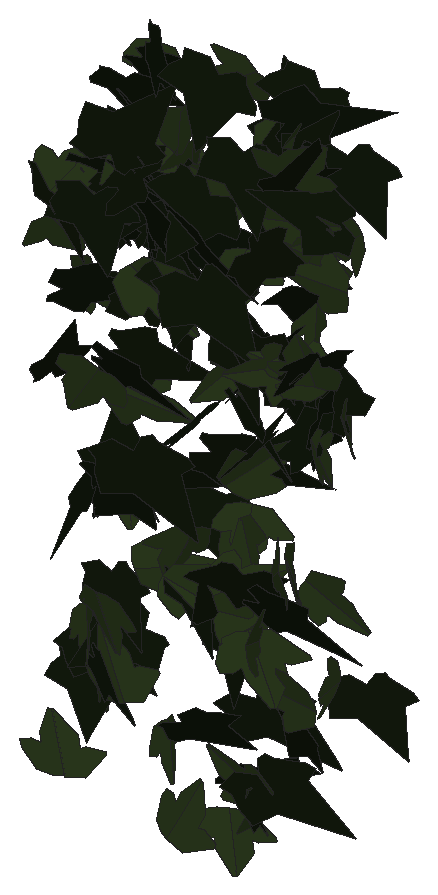
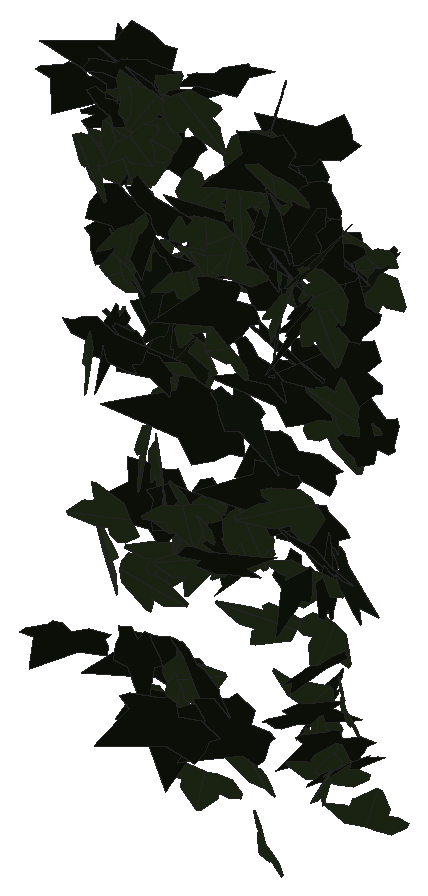
# SketchUp Ruby script. Lengths in inches.
U = 1.inch
M = Sketchup.active_model
def pt(a) = Geom::Point3d.new(a.map { |v| v * U })
def face(e, loops, mat)
  f = e.add_face(loops[0].map { |a| pt(a) })
  loops[1..].each { |l| e.add_face(l.map { |a| pt(a) }).erase! }
  f.material = f.back_material = mat if mat
  f
end
# faces: each face lists its corners as indices into pts; further lists are holes
def faces(e, pts, list, mat = nil) = list.each { |f| face(e, (f[0].is_a?(Array) ? f : [f]).map { |l| l.map { |i| pts[i] } }, mat) }
# xy, xz, yz: faces in a plane at the given z, y or x. An outline is a flat list of corners, or four numbers for a rectangle; further outlines are holes
def ring(l) = l.size == 4 ? [[l[0], l[1]], [l[2], l[1]], [l[2], l[3]], [l[0], l[3]]] : l.each_slice(2).to_a
def flat(e, list, mat, &to3) = list.each { |f| face(e, (f[0].is_a?(Array) ? f : [f]).map { |l| ring(l).map { |u, v| to3.(u, v) } }, mat) }
def xy(e, z, list, mat = nil) = flat(e, list, mat) { |x, y| [x, y, z] }
def xz(e, y, list, mat = nil) = flat(e, list, mat) { |x, z| [x, y, z] }
def yz(e, x, list, mat = nil) = flat(e, list, mat) { |y, z| [x, y, z] }
def lines(e, pts, list) = list.each { |a, b| e.add_line(pt(pts[a]), pt(pts[b])) }
# prism: a flat outline (further loops are holes) pulled along v
def prism(e, loops, v, mat = nil)
  f = face(e, loops, mat); d = Geom::Vector3d.new(v.map { |x| x * U })
  f.pushpull(f.normal.samedirection?(d) ? d.length : -d.length)
end
def box(e, o, s, mat = nil) = prism(e, [[o, [o[0] + s[0], o[1], o[2]], [o[0] + s[0], o[1] + s[1], o[2]], [o[0], o[1] + s[1], o[2]]]], [0, 0, s[2]], mat)
def at(x, y, z, deg = 0) = Geom::Transformation.translation(pt([x, y, z])) * Geom::Transformation.rotation(ORIGIN, Z_AXIS, deg.degrees)
def axes(o, x, y, z) = Geom::Transformation.new([*x, 0, *y, 0, *z, 0, *pt(o).to_a, 1])
def part(name) = M.definitions.add(name)
# library, detail: a bought-in or finely detailed component or shape, given as its bounding box
def library(name, o, s) = part(name).tap { |d| box(d.entities, o, s) }
def detail(e, o, s) = box(e.add_group.entities, o, s)
def put(e, d, t, mat = nil) = e.add_instance(d, t).tap { |i| i.material = mat if mat }
def group(e, t, mat = nil) = e.add_group.tap { |g| g.transformation = t; g.material = mat if mat }.entities
root = M.entities
M.materials.add("1026 AP 7946 SUNNY SIDE UP").color = [254, 231, 186]
M.materials.add("efeu1").color = [18, 25, 13]
M.materials.add("efeu2").color = [43, 57, 29]
c1 = part("ivyleaf_9")
p = [[1.54,2.16,1.25],[1.36,2.04,1.19],[-0.21,0.99,0.68],[-0.71,1.11,0.82],[-0.85,0.86,0.67],[-0.8,0.17,0.21],
  [-0.9,-0.01,0.1],[-0.67,-0.16,-0.02],[-0.08,-0.08,-0.05],[-0.03,-0.6,-0.4],[0.65,-0.88,-0.66],[0.83,-0.6,-0.49],
  [1.29,-0.42,-0.43],[1.8125,-0.07,-0.26],[1.21,0.44,0.15]]
faces(c1.entities,p,[[0,1,2,3,4,5,6,7,8,9,10,11,12,13,14]],"efeu1")
c2 = part("ivyleaf_10")
p = [[0,0.5,-0.03],[-0.0625,2.02,-0.43],[-0.19,2.01,-0.46],[-0.54,1.05,-0.29],[-0.52,0.625,-0.18],[-0.83,0.76,-0.28],
  [-1.16,0.64,-0.33],[-1.15,0.33,-0.24],[-0.77,-0.39,0.02],[-0.3,-0.51,0.16],[0.04,-0.48,0.23],[-0.02,2.01,-0.4375],
  [-0.06,2.01,-0.43],[0.04,-0.49,0.23],[0.67,-0.49,0.14],[1.38,0.36,-0.2],[1.375,0.51,-0.24],[0.81,0.65,-0.19],
  [0.62,0.59,-0.15],[0.6,1.09,-0.28],[0.5,1.23,-0.31]]
faces(c2.entities,p,[[0,1,2,3,4,5,6,7,8,9,10],[11,12,0,13,14,15,16,17,18,19,20]],"efeu2")
put(root,c1,axes([131.8,211.0625,274.17],[0.20977,0.25141,0.15948],[-0.19832,-0.10338,0.28698],[0.41845,-0.17502,0.05607]),"1026 AP 7946 SUNNY SIDE UP")
put(root,c2,axes([131.75,212.14,277.14],[-0.34587,0.07904,-0.20582],[0.25115,-0.13201,-0.23521],[-0.22694,-0.26655,0.05338]),"1026 AP 7946 SUNNY SIDE UP")
put(root,c1,axes([131.69,211.18,276.95],[0.1745,-0.32235,0.06334],[0.00781,-0.06517,-0.35119],[0.51649,0.10989,-0.01609]),"1026 AP 7946 SUNNY SIDE UP")
put(root,c2,axes([131.96,211.03,268.16],[0.45955,0.14826,0.03924],[-0.07352,0.01018,0.33625],[0.22885,-0.29445,0.02922]),"1026 AP 7946 SUNNY SIDE UP")
put(root,c2,axes([131.58,211.93,275.12],[0.00813,-0.00522,0.33783],[0.50626,-0.06254,-0.00662],[0.09847,0.32198,0.00615]),"1026 AP 7946 SUNNY SIDE UP")
put(root,c2,axes([131.96,210.88,276.61],[-0.22401,-0.24818,-0.19154],[0.17393,0.14883,-0.29333],[0.45411,-0.17943,0.01786]),"1026 AP 7946 SUNNY SIDE UP")
put(root,c1,axes([131.93,211.68,269.27],[-0.11331,-0.31358,0.02304],[0.00257,-0.02514,-0.33154],[0.49453,-0.07172,0.007]),"1026 AP 7946 SUNNY SIDE UP")
put(root,c2,axes([132.12,211.84,276.39],[-0.2045,-0.2943,0.06603],[-0.01394,-0.06786,-0.3313],[0.47397,-0.12898,0.01875]),"1026 AP 7946 SUNNY SIDE UP")
put(root,c1,axes([132.0625,211.5,272.28],[-0.34976,0.10596,-0.2904],[0.35323,-0.17612,-0.25131],[-0.31669,-0.31346,0.04042]),"1026 AP 7946 SUNNY SIDE UP")
put(root,c2,axes([132.07,211.7,269.17],[0.13469,-0.04751,-0.32807],[0.02732,0.32947,-0.04394],[0.50512,-0.00515,0.08986]),"1026 AP 7946 SUNNY SIDE UP")
put(root,c1,axes([131.98,211.6875,276.33],[0.50369,-0.15543,0.11191],[-0.12676,0.08328,0.36519],[-0.27076,-0.32813,0.03721]),"1026 AP 7946 SUNNY SIDE UP")
put(root,c1,axes([132,211.89,271.93],[0.04023,0.15172,0.30183],[-0.1497,-0.27707,0.15521],[0.49546,-0.09603,0.02239]),"1026 AP 7946 SUNNY SIDE UP")
put(root,c2,axes([131.875,211.1,277.09],[0.43761,0.04456,-0.16717],[0.22882,0.09467,0.28402],[0.13361,-0.30807,0.06109]),"1026 AP 7946 SUNNY SIDE UP")
put(root,c2,axes([132.11,211.7,269.12],[0.42989,0.18068,0.01962],[-0.0551,0.02054,0.33563],[0.28015,-0.27322,0.03591]),"1026 AP 7946 SUNNY SIDE UP")
put(root,c2,axes([131.88,211.59,270.18],[0.24733,-0.12321,0.26108],[0.29901,-0.16887,-0.20658],[0.32834,0.24659,-0.00854]),"1026 AP 7946 SUNNY SIDE UP")
put(root,c1,axes([132.18,212.23,277.25],[0.12672,-0.30585,-0.08111],[0.0579,-0.06981,0.32494],[-0.49254,-0.0869,0.01733]),"1026 AP 7946 SUNNY SIDE UP")
put(root,c1,axes([131.89,211.75,269.78],[0.07443,-0.18799,-0.26741],[0.09615,0.26182,-0.18308],[0.4933,-0.02267,0.07603]),"1026 AP 7946 SUNNY SIDE UP")
put(root,c1,axes([131.9,211.23,275.375],[0.28457,0.11751,0.29411],[0.41075,0.11664,-0.21989],[-0.25691,0.31666,-0.02579]),"1026 AP 7946 SUNNY SIDE UP")
put(root,c1,axes([132.42,211.77,272.5625],[-0.46411,0.12535,-0.06044],[-0.0735,0.04155,0.32998],[0.20534,0.29819,-0.01849]),"1026 AP 7946 SUNNY SIDE UP")
put(root,c1,axes([132.33,211.85,277.1],[0.34853,0.00144,0.2401],[-0.35863,0.06745,0.22344],[-0.07533,-0.31447,0.0471]),"1026 AP 7946 SUNNY SIDE UP")
put(root,c2,axes([132.54,211.03,274.33],[-0.49408,-0.03623,0.16001],[-0.23489,-0.05466,-0.32436],[0.08877,-0.34632,0.03236]),"1026 AP 7946 SUNNY SIDE UP")
put(root,c2,axes([132.35,211.7,269.33],[-0.4231,0.19063,0.03773],[0.06763,-0.0006,0.3388],[0.29732,0.27142,-0.02337]),"1026 AP 7946 SUNNY SIDE UP")
put(root,c1,axes([132.24,211.99,276.53],[0.23175,-0.20854,-0.26088],[-0.22103,0.20925,-0.26182],[0.46448,0.20363,0.00558]),"1026 AP 7946 SUNNY SIDE UP")
put(root,c1,axes([132.01,212.22,277.96],[0.36104,-0.19128,0.11563],[0.11208,-0.09098,-0.30751],[0.33113,0.23935,-0.02198]),"1026 AP 7946 SUNNY SIDE UP")
put(root,c1,axes([132.4375,212.08,276.42],[-0.1331,-0.1509,0.27183],[-0.19324,-0.2345,-0.17957],[0.43843,-0.14917,0.00338]),"1026 AP 7946 SUNNY SIDE UP")
put(root,c1,axes([132.39,211.92,278.47],[0.43253,0.13542,-0.12739],[-0.1516,-0.08445,-0.31476],[-0.24625,0.28985,-0.02998]),"1026 AP 7946 SUNNY SIDE UP")
put(root,c1,axes([132.6,211.95,270.02],[-0.36249,-0.19367,0.19789],[-0.19346,-0.15224,-0.30937],[0.38417,-0.25941,0.03093]),"1026 AP 7946 SUNNY SIDE UP")
put(root,c1,axes([132.26,211.76,270.83],[0.05408,-0.31384,-0.08522],[-0.00413,0.08112,-0.32472],[0.50961,0.03396,0.00641]),"1026 AP 7946 SUNNY SIDE UP")
put(root,c1,axes([132.43,211.96,272.34],[0.37578,-0.08418,-0.21747],[-0.31577,0.06371,-0.2606],[0.16581,0.31211,-0.00343]),"1026 AP 7946 SUNNY SIDE UP")
put(root,c2,axes([132.31,211.91,272.31],[0.47828,0.0842,0.08091],[0.1293,-0.0055,-0.32403],[-0.12599,0.31398,-0.02541]),"1026 AP 7946 SUNNY SIDE UP")
put(root,c1,axes([132.08,211.36,277.11],[0.40822,0.02408,0.25176],[0.38563,-0.03881,-0.26485],[0.01449,0.35433,-0.04401]),"1026 AP 7946 SUNNY SIDE UP")
put(root,c1,axes([132.6,212.0625,277.875],[0.04334,0.1272,0.34532],[0.11939,0.32576,-0.13216],[-0.54987,0.08075,-0.00148]),"1026 AP 7946 SUNNY SIDE UP")
put(root,c2,axes([132.55,212.15,276.6875],[-0.06651,0.30731,0.06583],[-0.03836,0.05931,-0.31881],[-0.4915,-0.04622,0.01597]),"1026 AP 7946 SUNNY SIDE UP")
put(root,c2,axes([132.3,212.13,273.48],[-0.20865,-0.08208,-0.31553],[0.45198,0.10785,-0.15768],[0.20882,-0.31544,0.02601]),"1026 AP 7946 SUNNY SIDE UP")
put(root,c2,axes([132.51,212.39,278.7],[0.47088,-0.05357,0.05829],[0.07814,-0.04333,-0.31177],[0.09483,0.30173,-0.03256]),"1026 AP 7946 SUNNY SIDE UP")
put(root,c1,axes([132.89,211.16,272.71],[0.26954,0.06338,-0.28984],[-0.41888,-0.09166,-0.18878],[-0.17514,0.31676,0.00545]),"1026 AP 7946 SUNNY SIDE UP")
put(root,c2,axes([132.69,211.01,270.87],[-0.47015,0.1397,-0.05002],[0.0485,-0.05001,-0.33869],[-0.22786,-0.29889,0.03111]),"1026 AP 7946 SUNNY SIDE UP")
put(root,c1,axes([132.58,210.96,277.125],[-0.30018,-0.17419,-0.21679],[0.31893,0.07984,-0.2584],[0.28594,-0.27191,0.06062]),"1026 AP 7946 SUNNY SIDE UP")
put(root,c1,axes([132.62,210.98,269.95],[0.30322,-0.20065,-0.14868],[-0.17539,0.09108,-0.28573],[0.34564,0.22224,-0.01456]),"1026 AP 7946 SUNNY SIDE UP")
put(root,c1,axes([133.21,211.16,277.58],[-0.4063,0.29603,0.15865],[-0.18235,0.10071,-0.40371],[-0.4907,-0.28254,0.01866]),"1026 AP 7946 SUNNY SIDE UP")
put(root,c1,axes([132.56,211.33,278.02],[0.51663,-0.15607,-0.06305],[-0.10989,-0.00724,-0.37292],[0.23905,0.33397,-0.03517]),"1026 AP 7946 SUNNY SIDE UP")
put(root,c2,axes([132.96,211.08,269.65],[0.50481,-0.02514,0.19623],[-0.29109,0.05976,0.32968],[-0.08164,-0.36856,0.03785]),"1026 AP 7946 SUNNY SIDE UP")
put(root,c2,axes([132.58,212.5,268.2],[0.27802,-0.11661,0.25702],[0.30993,-0.1546,-0.21867],[0.30377,0.26446,-0.01213]),"1026 AP 7946 SUNNY SIDE UP")
put(root,c2,axes([132.91,211.61,277.84],[0.42103,0.1767,-0.20197],[-0.23811,-0.12762,-0.33062],[-0.34134,0.30699,-0.01849]),"1026 AP 7946 SUNNY SIDE UP")
put(root,c1,axes([132.99,211.61,276.53],[0.21354,-0.10578,-0.29384],[-0.39787,0.13295,-0.1745],[0.26395,0.28598,-0.0253]),"1026 AP 7946 SUNNY SIDE UP")
put(root,c1,axes([133.05,211.76,277.09],[-0.45363,0.09313,-0.15725],[0.20853,-0.08437,-0.31068],[-0.18965,-0.31555,0.03452]),"1026 AP 7946 SUNNY SIDE UP")
put(root,c1,axes([132.6,212.1,278.77],[0.48316,0.02468,0.12688],[0.19574,-0.01927,-0.31645],[-0.02467,0.33042,-0.02598]),"1026 AP 7946 SUNNY SIDE UP")
put(root,c1,axes([132.98,211.49,275.34],[-0.42218,0.22691,0.07167],[0.10808,-0.02417,0.36106],[0.35658,0.27598,-0.02458]),"1026 AP 7946 SUNNY SIDE UP")
put(root,c1,axes([133.1,211.56,279.41],[0.25252,-0.17133,-0.27959],[-0.35031,0.15745,-0.23814],[0.36148,0.27227,-0.03547]),"1026 AP 7946 SUNNY SIDE UP")
put(root,c1,axes([133.46,211.78,277.49],[0.2133,0.02382,-0.29051],[-0.43234,-0.06358,-0.1421],[-0.10626,0.30653,-0.00502]),"1026 AP 7946 SUNNY SIDE UP")
put(root,c1,axes([132.85,211.26,274.73],[0.24395,0.01143,-0.31631],[0.2866,0.27356,0.10695],[0.38906,-0.20868,0.11955]),"1026 AP 7946 SUNNY SIDE UP")
put(root,c1,axes([133.09,210.73,278.15],[-0.19545,-0.04257,0.39666],[0.53628,0.18024,0.13493],[-0.28962,0.36249,-0.01783]),"1026 AP 7946 SUNNY SIDE UP")
put(root,c1,axes([132.9,210.86,274.75],[0.44134,-0.10229,0.15805],[0.21135,-0.07932,-0.30711],[0.19959,0.31017,-0.02428]),"1026 AP 7946 SUNNY SIDE UP")
put(root,c2,axes([132.95,211.74,271.22],[0.17155,-0.01783,-0.31849],[0.46861,0.09473,0.1033],[0.13173,-0.31376,0.04728]),"1026 AP 7946 SUNNY SIDE UP")
put(root,c1,axes([133.2,211.92,275.45],[-0.25039,-0.04522,-0.29385],[0.45253,-0.00152,-0.16543],[0.03258,-0.32645,0.03953]),"1026 AP 7946 SUNNY SIDE UP")
put(root,c2,axes([133.52,211.88,277.86],[-0.0774,-0.32256,-0.0814],[0.03281,0.07486,-0.33558],[0.52049,-0.05268,0.00905]),"1026 AP 7946 SUNNY SIDE UP")
put(root,c1,axes([133.23,211.28,276.93],[-0.0264,-0.02253,0.38097],[0.13979,-0.35975,-0.02052],[0.56575,0.08784,0.02285]),"1026 AP 7946 SUNNY SIDE UP")
put(root,c1,axes([133.2,211.26,272.99],[0.11913,0.14487,-0.30119],[0.18439,0.2689,0.16967],[0.48002,-0.13924,0.00957]),"1026 AP 7946 SUNNY SIDE UP")
put(root,c2,axes([133.6,211.53,278.53],[-0.26706,-0.29275,-0.01958],[0.03804,0.00599,-0.34815],[0.45956,-0.17062,0.01744]),"1026 AP 7946 SUNNY SIDE UP")
put(root,c2,axes([133.58,212.14,276.82],[0.5438,0.09829,0.05112],[-0.08879,0.02004,0.36881],[0.14817,-0.34873,0.0334]),"1026 AP 7946 SUNNY SIDE UP")
put(root,c1,axes([134.01,212.11,272.03],[-0.42831,-0.17347,-0.09606],[-0.1472,-0.02406,0.33122],[-0.27162,0.28658,-0.02804]),"1026 AP 7946 SUNNY SIDE UP")
put(root,c1,axes([133.36,210.89,273.46],[-0.16243,-0.15883,-0.35347],[0.42834,0.21407,-0.18581],[0.41041,-0.28628,0.05404]),"1026 AP 7946 SUNNY SIDE UP")
put(root,c1,axes([133.49,212.12,276.33],[0.05118,0.09663,-0.32384],[0.02958,0.31537,0.10355],[0.51709,-0.0276,0.02613]),"1026 AP 7946 SUNNY SIDE UP")
put(root,c2,axes([133.92,212.22,277.37],[-0.47357,-0.07052,0.03676],[-0.04331,-0.03978,-0.31716],[0.11679,-0.30071,0.03145]),"1026 AP 7946 SUNNY SIDE UP")
put(root,c1,axes([133.48,211.82,277.125],[-0.02765,0.04124,0.34155],[0.52011,-0.04289,0.02334],[0.07127,0.32899,-0.03779]),"1026 AP 7946 SUNNY SIDE UP")
put(root,c2,axes([133.43,210.93,276.17],[0.34469,0.06149,0.32254],[0.48343,0.05927,-0.23367],[-0.13212,0.37729,-0.01354]),"1026 AP 7946 SUNNY SIDE UP")
put(root,c1,axes([133.47,211.38,276.39],[0.13907,-0.02312,-0.3083],[0.45938,0.07762,0.08326],[0.10738,-0.30213,0.04308]),"1026 AP 7946 SUNNY SIDE UP")
put(root,c2,axes([133.56,212.13,275.57],[0.3357,-0.05918,0.29437],[0.40924,-0.1224,-0.22689],[0.20863,0.33532,-0.02859]),"1026 AP 7946 SUNNY SIDE UP")
put(root,c2,axes([133.99,211.21,272.28],[-0.19364,-0.31747,0.0972],[-0.03192,-0.09516,-0.35102],[0.5206,-0.12392,0.01463]),"1026 AP 7946 SUNNY SIDE UP")
put(root,c1,axes([134.17,211.22,274.125],[-0.2252,0.29588,-0.07605],[0.03176,-0.07403,-0.33879],[-0.4791,-0.14399,0.01329]),"1026 AP 7946 SUNNY SIDE UP")
put(root,c1,axes([133.77,211.45,269.21],[0.38707,0.17433,0.13301],[0.19002,0.05018,-0.30924],[-0.28216,0.27293,-0.0258]),"1026 AP 7946 SUNNY SIDE UP")
put(root,c2,axes([134.31,212.13,279.14],[-0.34314,-0.01104,0.23554],[-0.35282,-0.0526,-0.2235],[0.07168,-0.31171,0.02749]),"1026 AP 7946 SUNNY SIDE UP")
put(root,c1,axes([134.02,211.22,276.31],[-0.21853,-0.30988,0.02026],[0.00597,-0.02516,-0.34973],[0.48838,-0.13835,0.01334]),"1026 AP 7946 SUNNY SIDE UP")
put(root,c1,axes([133.98,212.29,270.45],[-0.34,-0.01552,-0.3119],[0.47348,-0.05308,-0.21912],[-0.05394,-0.36816,0.04253]),"1026 AP 7946 SUNNY SIDE UP")
put(root,c2,axes([134.31,211.86,277.53],[-0.16145,-0.15407,-0.29231],[-0.28419,-0.21819,0.18874],[-0.41923,0.20724,-0.01537]),"1026 AP 7946 SUNNY SIDE UP")
put(root,c1,axes([133.96,211.27,271.53],[0.11072,-0.32091,0.05876],[0.01375,-0.05834,-0.33878],[0.51283,0.07085,-0.0036]),"1026 AP 7946 SUNNY SIDE UP")
put(root,c1,axes([134.23,211.34,277.55],[-0.32508,-0.28044,0.07865],[-0.04473,-0.07568,-0.35869],[0.45548,-0.20758,0.02091]),"1026 AP 7946 SUNNY SIDE UP")
put(root,c2,axes([134.03,210.93,271.67],[0.09576,0.19501,0.25172],[0.13778,0.22713,-0.20887],[-0.47044,0.10622,-0.00994]),"1026 AP 7946 SUNNY SIDE UP")
put(root,c2,axes([134.12,210.8125,268],[0.50509,-0.1841,-0.06742],[0.11388,-0.00261,0.37986],[-0.28474,-0.3276,0.03233]),"1026 AP 7946 SUNNY SIDE UP")
put(root,c1,axes([134.3,211.47,279.37],[-0.27356,-0.30547,0.00866],[0.01737,-0.01794,-0.36176],[0.48028,-0.17335,0.01802]),"1026 AP 7946 SUNNY SIDE UP")
put(root,c2,axes([134.4,211.93,276.34],[0.27352,0.26767,-0.10423],[-0.06686,-0.0947,-0.32905],[-0.44582,0.17843,-0.0146]),"1026 AP 7946 SUNNY SIDE UP")
put(root,c1,axes([134.13,210.97,277.18],[0.38563,-0.22039,0.20023],[0.19188,-0.1557,-0.33923],[0.42176,0.27234,-0.02875]),"1026 AP 7946 SUNNY SIDE UP")
put(root,c2,axes([134.5625,211.84,272.5],[0.39264,0.19971,-0.05101],[-0.03771,-0.05086,-0.32873],[-0.32176,0.24966,-0.02371]),"1026 AP 7946 SUNNY SIDE UP")
put(root,c1,axes([134.43,212.22,269.4375],[-0.05868,-0.07936,-0.37433],[0.32587,0.29825,-0.0874],[0.48478,-0.2101,0.01344]),"1026 AP 7946 SUNNY SIDE UP")
put(root,c1,axes([134.52,210.82,276.53],[-0.03717,-0.28285,-0.28991],[0.1263,0.27114,-0.28777],[0.61272,-0.07305,0.04173]),"1026 AP 7946 SUNNY SIDE UP")
put(root,c1,axes([135.07,211.93,277.07],[0.0276,0.0368,0.34533],[-0.26555,0.29126,-0.02214],[-0.45859,-0.16644,0.0336]),"1026 AP 7946 SUNNY SIDE UP")
put(root,c2,axes([134.875,211.22,275.25],[0.14479,0.15883,-0.3576],[-0.23769,-0.31372,-0.19054],[-0.55257,0.17657,-0.01174]),"1026 AP 7946 SUNNY SIDE UP")
put(root,c2,axes([134.62,211.32,268.04],[0.48517,0.1111,0.06631],[0.11188,-0.01044,-0.33616],[-0.16747,0.31489,-0.03247]),"1026 AP 7946 SUNNY SIDE UP")
put(root,c2,axes([134.57,211.64,272.375],[0.36525,-0.07219,0.23401],[0.31776,-0.10959,-0.24897],[0.19987,0.30616,-0.03182]),"1026 AP 7946 SUNNY SIDE UP")
put(root,c1,axes([135.125,210.95,272.16],[0.13406,0.22258,-0.29579],[-0.13819,-0.27486,-0.24693],[-0.5559,0.12201,-0.00995]),"1026 AP 7946 SUNNY SIDE UP")
put(root,c1,axes([134.49,211.23,273.73],[0.20701,0.11424,-0.37222],[0.36929,0.27645,0.1795],[0.46885,-0.26818,0.02296]),"1026 AP 7946 SUNNY SIDE UP")
put(root,c1,axes([135.07,211.43,268.97],[0.26522,0.31683,-0.06783],[-0.02647,-0.06759,-0.36976],[-0.50872,0.16869,-0.01612]),"1026 AP 7946 SUNNY SIDE UP")
put(root,c1,axes([134.87,211.14,275.5625],[0.09802,-0.33224,0.03041],[0.00066,-0.03187,-0.34839],[0.52475,0.0621,-0.00524]),"1026 AP 7946 SUNNY SIDE UP")
put(root,c1,axes([134.87,211.34,268.54],[0.00591,-0.18591,0.28815],[0.08014,-0.27723,-0.19144],[0.52338,0.04455,0.02606]),"1026 AP 7946 SUNNY SIDE UP")
put(root,c2,axes([134.95,210.93,271.21],[0.06837,0.05505,-0.38077],[0.26382,0.32997,0.07283],[0.52558,-0.17279,0.01298]),"1026 AP 7946 SUNNY SIDE UP")
put(root,c2,axes([135.11,212.3,278.41],[0.16726,0.24497,-0.17112],[-0.1194,-0.14954,-0.27586],[-0.45109,0.13041,0.00957]),"1026 AP 7946 SUNNY SIDE UP")
put(root,c2,axes([134.85,210.98,271.88],[0.11505,0.05302,-0.38141],[0.37554,0.28409,0.09212],[0.45318,-0.24888,0.02049]),"1026 AP 7946 SUNNY SIDE UP")
put(root,c2,axes([135.5,210.77,269.0625],[-0.26182,0.03199,-0.28213],[-0.40387,0.0989,0.17325],[0.1584,0.30503,-0.02459]),"1026 AP 7946 SUNNY SIDE UP")
put(root,c1,axes([134.91,211.77,275.4375],[0.1928,-0.26021,0.17437],[0.10531,-0.15715,-0.2972],[0.4779,0.13961,-0.00486]),"1026 AP 7946 SUNNY SIDE UP")
put(root,c1,axes([135.11,211.03,278.63],[-0.09455,-0.34206,-0.08695],[0.01633,0.0819,-0.35729],[0.55303,-0.0609,-0.00432]),"1026 AP 7946 SUNNY SIDE UP")
put(root,c1,axes([135.6,210.97,275.48],[0.03532,0.00823,0.35797],[-0.40622,0.23327,0.01288],[-0.36551,-0.25846,0.02028]),"1026 AP 7946 SUNNY SIDE UP")
put(root,c1,axes([135.49,211.35,275.71],[-0.25619,0.25185,-0.24221],[0.16031,-0.21483,-0.30924],[-0.51909,-0.19064,0.02404]),"1026 AP 7946 SUNNY SIDE UP")
put(root,c1,axes([135.68,211.59,278.89],[-0.54629,0.11443,-0.12538],[-0.16632,0.06863,0.37592],[0.20428,0.36189,-0.02924]),"1026 AP 7946 SUNNY SIDE UP")
put(root,c2,axes([135.33,212.1,276.82],[0.0994,0.32566,-0.06244],[-0.00896,-0.0625,-0.34207],[-0.52133,0.06317,-0.00602]),"1026 AP 7946 SUNNY SIDE UP")
put(root,c2,axes([135.22,211.73,278.76],[0.35384,0.1962,0.11896],[0.14354,0.06926,-0.30707],[-0.32696,0.24273,-0.00607]),"1026 AP 7946 SUNNY SIDE UP")
put(root,c1,axes([135.14,210.94,274.85],[0.34096,-0.26532,0.0034],[-0.01782,-0.01546,-0.35258],[0.41689,0.21634,-0.01785]),"1026 AP 7946 SUNNY SIDE UP")
put(root,c2,axes([135.4375,211.07,268.64],[-0.13749,-0.24111,-0.23572],[-0.07315,-0.22397,0.26171],[-0.51602,0.09599,0.0257]),"1026 AP 7946 SUNNY SIDE UP")
put(root,c1,axes([135.19,211.91,274.84],[-0.19847,-0.0441,-0.31139],[0.47163,0.04255,-0.13529],[0.0888,-0.32455,0.02261]),"1026 AP 7946 SUNNY SIDE UP")
put(root,c2,axes([135.3,210.77,273.83],[-0.10643,-0.24465,0.31492],[0.10362,0.30011,0.26304],[-0.6086,0.09388,-0.01029]),"1026 AP 7946 SUNNY SIDE UP")
put(root,c1,axes([135.54,210.52,274.34],[-0.24404,0.24583,-0.22232],[-0.15172,0.19544,0.30006],[0.49299,0.18184,-0.01771]),"1026 AP 7946 SUNNY SIDE UP")
put(root,c2,axes([135.63,210.57,271.44],[-0.03558,0.13024,0.33456],[-0.27197,0.27789,-0.12589],[-0.47701,-0.16815,0.04682]),"1026 AP 7946 SUNNY SIDE UP")
put(root,c2,axes([135.52,211.98,278.86],[-0.02905,0.01692,-0.34828],[-0.07769,-0.33518,-0.01646],[-0.5267,0.04851,0.02164]),"1026 AP 7946 SUNNY SIDE UP")
put(root,c1,axes([135.56,212.0625,279.35],[-0.39596,-0.22327,-0.02157],[0.05216,-0.00786,-0.34556],[0.34855,-0.25246,0.02721]),"1026 AP 7946 SUNNY SIDE UP")
put(root,c2,axes([135.34,210.95,271.16],[0.45153,0.23448,0.1024],[0.14613,0.04086,-0.38073],[-0.37197,0.30068,-0.02526]),"1026 AP 7946 SUNNY SIDE UP")
put(root,c1,axes([135.7,211.45,269.85],[0.27756,-0.0169,-0.28082],[-0.42814,0.01291,-0.18246],[0.0315,0.32442,-0.00547]),"1026 AP 7946 SUNNY SIDE UP")
put(root,c2,axes([135.77,211.05,275.58],[0.03176,-0.01052,-0.36925],[-0.34401,-0.28472,-0.00576],[-0.44661,0.21856,-0.02182]),"1026 AP 7946 SUNNY SIDE UP")
put(root,c2,axes([135.9,210.82,272.52],[-0.18558,0.16747,0.29719],[-0.35949,0.18084,-0.20413],[-0.38014,-0.25278,0.04797]),"1026 AP 7946 SUNNY SIDE UP")
put(root,c1,axes([136.12,211.88,274.65],[-0.16287,0.08117,0.32545],[-0.45615,0.12753,-0.13119],[-0.23289,-0.30655,0.02936]),"1026 AP 7946 SUNNY SIDE UP")
put(root,c1,axes([135.61,210.61,277.49],[0.06451,-0.0052,-0.34926],[-0.14108,0.32912,-0.01446],[0.51408,0.09098,0.03986]),"1026 AP 7946 SUNNY SIDE UP")
put(root,c2,axes([136.14,210.95,270.55],[0.03459,-0.01525,-0.35097],[-0.46904,0.16443,-0.02647],[0.25962,0.29909,-0.00106]),"1026 AP 7946 SUNNY SIDE UP")
put(root,c1,axes([135.92,211.34,276.73],[0.11321,0.32301,-0.08276],[-0.02092,-0.08121,-0.34137],[-0.52367,0.07308,-0.00425]),"1026 AP 7946 SUNNY SIDE UP")
put(root,c1,axes([135.47,211.56,279.04],[0.15945,0.04124,0.38217],[0.57317,0.07058,-0.1104],[-0.12448,0.37781,-0.01878]),"1026 AP 7946 SUNNY SIDE UP")
put(root,c2,axes([135.69,211.78,276.04],[0.34267,-0.15284,0.22013],[0.24473,-0.14994,-0.27379],[0.33418,0.26653,-0.02522]),"1026 AP 7946 SUNNY SIDE UP")
put(root,c2,axes([135.74,211.24,278.47],[-0.43655,-0.14665,0.15204],[0.20622,0.06948,0.32387],[-0.25516,0.30705,0.00163]),"1026 AP 7946 SUNNY SIDE UP")
put(root,c2,axes([135.54,211.18,277.71],[-0.17756,-0.03938,0.32303],[0.45695,0.11849,0.12375],[-0.19613,0.31172,-0.00412]),"1026 AP 7946 SUNNY SIDE UP")
put(root,c2,axes([136.13,211.21,275.45],[0.12586,0.17315,0.30573],[-0.25205,-0.24956,0.19373],[0.47635,-0.1778,0.02173]),"1026 AP 7946 SUNNY SIDE UP")
put(root,c1,axes([135.76,211.29,278.26],[0.36815,0.2341,0.17412],[-0.22212,-0.09496,0.3392],[0.39457,-0.27188,0.02849]),"1026 AP 7946 SUNNY SIDE UP")
put(root,c1,axes([136.24,211.15,274.59],[-0.38168,0.24591,0.04468],[-0.07536,0.0115,-0.3549],[-0.38496,-0.24607,0.02518]),"1026 AP 7946 SUNNY SIDE UP")
put(root,c2,axes([136.05,210.86,272.69],[-0.24914,0.27394,0.13141],[-0.14689,0.09074,-0.32371],[-0.45079,-0.18096,0.03286]),"1026 AP 7946 SUNNY SIDE UP")
put(root,c1,axes([135.5625,210.92,271.89],[0.51473,-0.05164,0.17172],[0.24885,-0.06292,-0.34003],[0.11666,0.36206,-0.03237]),"1026 AP 7946 SUNNY SIDE UP")
put(root,c1,axes([135.67,210.73,269.35],[0.06599,-0.10354,-0.36656],[0.28622,0.31703,-0.07119],[0.50654,-0.16565,0.08798]),"1026 AP 7946 SUNNY SIDE UP")
put(root,c1,axes([136.14,211.36,274.75],[0.07421,-0.05424,-0.36646],[-0.3932,0.2526,-0.07245],[0.40618,0.25444,-0.00318]),"1026 AP 7946 SUNNY SIDE UP")
put(root,c2,axes([136.02,211.28,277.16],[-0.4974,-0.11978,0.09843],[0.13352,0.04725,0.34846],[-0.20134,0.32725,-0.01208]),"1026 AP 7946 SUNNY SIDE UP")
put(root,c2,axes([136.27,211.8,274.58],[-0.18335,0.22998,0.22813],[-0.2261,0.17112,-0.26163],[-0.44662,-0.18104,0.03879]),"1026 AP 7946 SUNNY SIDE UP")
put(root,c2,axes([136.28,211.02,275.62],[-0.4816,-0.05417,-0.07303],[-0.11372,0.0042,0.32001],[-0.08149,0.31428,-0.01497]),"1026 AP 7946 SUNNY SIDE UP")
put(root,c1,axes([136.45,211.375,277.93],[-0.17843,-0.26441,-0.17818],[-0.1129,-0.15574,0.29548],[-0.48249,0.13423,-0.00325]),"1026 AP 7946 SUNNY SIDE UP")
put(root,c2,axes([135.86,211.67,271.875],[0.19247,0.00997,0.31271],[0.47342,0.03851,-0.12618],[-0.06201,0.32497,0.00729]),"1026 AP 7946 SUNNY SIDE UP")
put(root,c1,axes([136.43,211.01,275.97],[-0.07414,0.24695,-0.20383],[-0.00236,-0.20162,-0.25823],[-0.49893,-0.03574,0.03151]),"1026 AP 7946 SUNNY SIDE UP")
put(root,c2,axes([136.45,211.7,277.56],[0.30007,-0.18292,-0.2185],[-0.18827,0.17736,-0.26884],[0.39675,0.2225,0.03768]),"1026 AP 7946 SUNNY SIDE UP")
put(root,c2,axes([136.71,211.02,277.15],[-0.05409,0.08731,0.33285],[-0.52411,0.01461,-0.04061],[-0.03821,-0.3241,0.0858]),"1026 AP 7946 SUNNY SIDE UP")
put(root,c2,axes([136.41,211.01,274.55],[-0.13606,0.28623,0.10882],[-0.07517,0.09401,-0.30697],[-0.47292,-0.09729,0.01749]),"1026 AP 7946 SUNNY SIDE UP")
put(root,c1,axes([136.21,212.33,270.22],[-0.12006,-0.22225,-0.23446],[0.15881,0.20364,-0.23992],[0.47281,-0.12483,0.02105]),"1026 AP 7946 SUNNY SIDE UP")
put(root,c2,axes([136.62,211.0625,271],[0.129,-0.26721,-0.20707],[-0.13289,0.18207,-0.28598],[0.50721,0.11566,-0.02226]),"1026 AP 7946 SUNNY SIDE UP")
put(root,c1,axes([136.35,211.74,278.71],[-0.21592,-0.185,-0.26396],[0.27028,0.18935,-0.23561],[0.41541,-0.21936,0.0161]),"1026 AP 7946 SUNNY SIDE UP")
